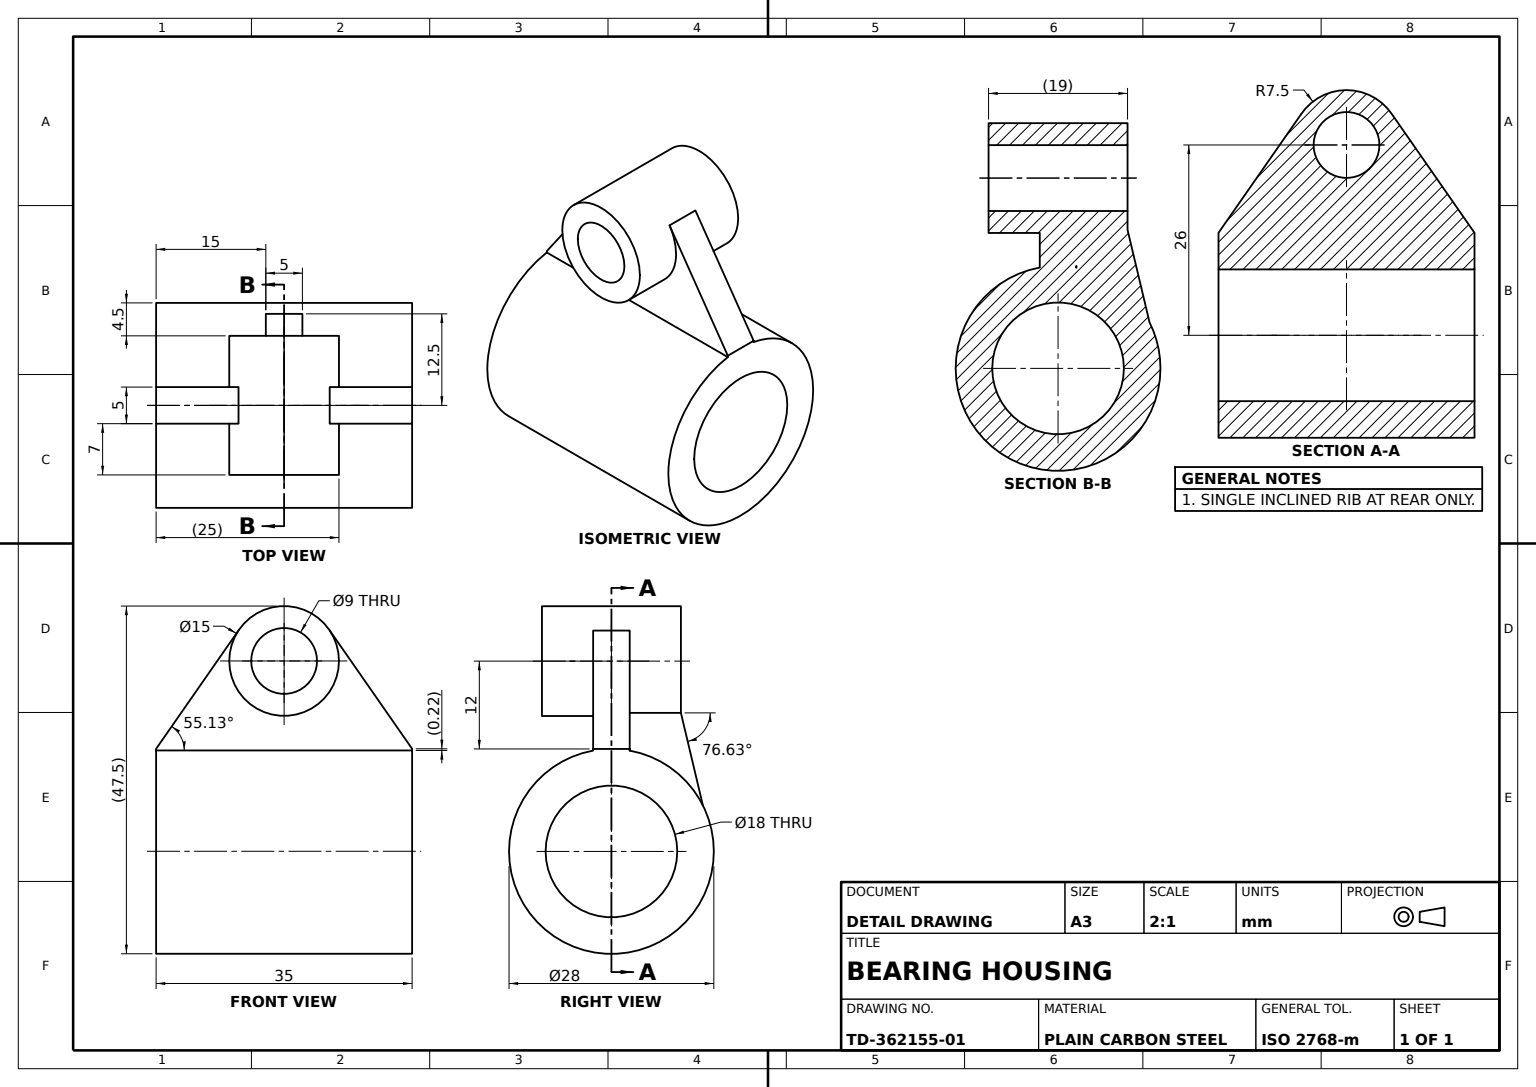
ISO-10303-21;
HEADER;
FILE_DESCRIPTION((''),'2;1');
FILE_NAME('','',(''),(''),'','','');
FILE_SCHEMA(('AUTOMOTIVE_DESIGN'));
ENDSEC;
DATA;
#1=APPLICATION_CONTEXT('');
#2=PRODUCT_CONTEXT('',#1,'mechanical');
#3=PRODUCT('','','',(#2));
#4=PRODUCT_DEFINITION_FORMATION('','',#3);
#5=PRODUCT_DEFINITION_CONTEXT('',#1,'design');
#6=PRODUCT_DEFINITION('','',#4,#5);
#7=PRODUCT_DEFINITION_SHAPE('','',#6);
#8=(LENGTH_UNIT()NAMED_UNIT(*)SI_UNIT(.MILLI.,.METRE.));
#9=(NAMED_UNIT(*)PLANE_ANGLE_UNIT()SI_UNIT($,.RADIAN.));
#10=(NAMED_UNIT(*)SI_UNIT($,.STERADIAN.)SOLID_ANGLE_UNIT());
#11=UNCERTAINTY_MEASURE_WITH_UNIT(LENGTH_MEASURE(1.E-05),#8,'distance_accuracy_value','');
#12=(GEOMETRIC_REPRESENTATION_CONTEXT(3)GLOBAL_UNCERTAINTY_ASSIGNED_CONTEXT((#11))GLOBAL_UNIT_ASSIGNED_CONTEXT((#8,#9,#10))REPRESENTATION_CONTEXT('',''));
#13=CARTESIAN_POINT('',(9.5,26.,-22.));
#14=VERTEX_POINT('',#13);
#15=CARTESIAN_POINT('',(9.5,26.,-13.));
#16=VERTEX_POINT('',#15);
#17=CARTESIAN_POINT('',(9.5,26.,-17.5));
#18=DIRECTION('',(1.,0.,0.));
#19=DIRECTION('',(0.,0.,-1.));
#20=AXIS2_PLACEMENT_3D('',#17,#18,#19);
#21=CIRCLE('',#20,4.5);
#22=EDGE_CURVE('',#14,#16,#21,.T.);
#23=ORIENTED_EDGE('',*,*,#22,.F.);
#24=EDGE_CURVE('',#16,#14,#21,.T.);
#25=ORIENTED_EDGE('',*,*,#24,.F.);
#26=EDGE_LOOP('',(#23,#25));
#27=FACE_BOUND('',#26,.T.);
#28=CARTESIAN_POINT('',(9.5,18.928932,-20.));
#29=VERTEX_POINT('',#28);
#30=CARTESIAN_POINT('',(9.5,18.928932,-15.));
#31=VERTEX_POINT('',#30);
#32=CARTESIAN_POINT('',(9.5,18.928932,-35.));
#33=DIRECTION('',(0.,0.,1.));
#34=VECTOR('',#33,1000.);
#35=LINE('',#32,#34);
#36=EDGE_CURVE('',#29,#31,#35,.T.);
#37=ORIENTED_EDGE('',*,*,#36,.F.);
#38=CARTESIAN_POINT('',(9.5,26.,-25.));
#39=VERTEX_POINT('',#38);
#40=CIRCLE('',#20,7.5);
#41=EDGE_CURVE('',#29,#39,#40,.T.);
#42=ORIENTED_EDGE('',*,*,#41,.T.);
#43=CARTESIAN_POINT('',(9.5,26.,-10.));
#44=VERTEX_POINT('',#43);
#45=EDGE_CURVE('',#39,#44,#40,.T.);
#46=ORIENTED_EDGE('',*,*,#45,.T.);
#47=EDGE_CURVE('',#44,#31,#40,.T.);
#48=ORIENTED_EDGE('',*,*,#47,.T.);
#49=EDGE_LOOP('',(#37,#42,#46,#48));
#50=FACE_OUTER_BOUND('',#49,.T.);
#51=PLANE('',#20);
#52=ADVANCED_FACE('',(#27,#50),#51,.T.);
#53=CARTESIAN_POINT('',(14.,0.,-35.));
#54=VERTEX_POINT('',#53);
#55=CARTESIAN_POINT('',(14.,0.,0.));
#56=VERTEX_POINT('',#55);
#57=LINE('',#53,#34);
#58=EDGE_CURVE('',#54,#56,#57,.T.);
#59=ORIENTED_EDGE('',*,*,#58,.T.);
#60=CARTESIAN_POINT('',(-14.,0.,0.));
#61=VERTEX_POINT('',#60);
#62=CARTESIAN_POINT('',(0.,0.,0.));
#63=AXIS2_PLACEMENT_3D('',#62,#33,#18);
#64=CIRCLE('',#63,14.);
#65=EDGE_CURVE('',#61,#56,#64,.T.);
#66=ORIENTED_EDGE('',*,*,#65,.F.);
#67=CARTESIAN_POINT('',(-14.,0.,-35.));
#68=VERTEX_POINT('',#67);
#69=LINE('',#67,#34);
#70=EDGE_CURVE('',#68,#61,#69,.T.);
#71=ORIENTED_EDGE('',*,*,#70,.F.);
#72=CARTESIAN_POINT('',(0.,0.,-35.));
#73=AXIS2_PLACEMENT_3D('',#72,#33,#18);
#74=CIRCLE('',#73,14.);
#75=EDGE_CURVE('',#68,#54,#74,.T.);
#76=ORIENTED_EDGE('',*,*,#75,.T.);
#77=EDGE_LOOP('',(#59,#66,#71,#76));
#78=FACE_OUTER_BOUND('',#77,.T.);
#79=CYLINDRICAL_SURFACE('',#73,14.);
#80=ADVANCED_FACE('',(#78),#79,.T.);
#81=CARTESIAN_POINT('',(2.5,26.,-25.));
#82=VERTEX_POINT('',#81);
#83=CARTESIAN_POINT('',(-2.5,26.,-25.));
#84=VECTOR('',#18,1000.);
#85=LINE('',#83,#84);
#86=EDGE_CURVE('',#82,#39,#85,.T.);
#87=ORIENTED_EDGE('',*,*,#86,.F.);
#88=CARTESIAN_POINT('',(2.5,30.172304,-23.732325));
#89=VERTEX_POINT('',#88);
#90=CARTESIAN_POINT('',(2.5,26.,-17.5));
#91=AXIS2_PLACEMENT_3D('',#90,#18,#19);
#92=CIRCLE('',#91,7.5);
#93=EDGE_CURVE('',#82,#89,#92,.T.);
#94=ORIENTED_EDGE('',*,*,#93,.T.);
#95=CARTESIAN_POINT('',(-2.5,30.172304,-23.732325));
#96=VERTEX_POINT('',#95);
#97=LINE('',#95,#84);
#98=EDGE_CURVE('',#96,#89,#97,.T.);
#99=ORIENTED_EDGE('',*,*,#98,.F.);
#100=VERTEX_POINT('',#83);
#101=CARTESIAN_POINT('',(-2.5,26.,-17.5));
#102=DIRECTION('',(-1.,0.,0.));
#103=AXIS2_PLACEMENT_3D('',#101,#102,#33);
#104=CIRCLE('',#103,7.5);
#105=EDGE_CURVE('',#96,#100,#104,.T.);
#106=ORIENTED_EDGE('',*,*,#105,.T.);
#107=CARTESIAN_POINT('',(-9.5,26.,-25.));
#108=VERTEX_POINT('',#107);
#109=EDGE_CURVE('',#108,#100,#85,.T.);
#110=ORIENTED_EDGE('',*,*,#109,.F.);
#111=CARTESIAN_POINT('',(-9.5,26.,-10.));
#112=VERTEX_POINT('',#111);
#113=CARTESIAN_POINT('',(-9.5,26.,-17.5));
#114=AXIS2_PLACEMENT_3D('',#113,#102,#33);
#115=CIRCLE('',#114,7.5);
#116=EDGE_CURVE('',#112,#108,#115,.T.);
#117=ORIENTED_EDGE('',*,*,#116,.F.);
#118=CARTESIAN_POINT('',(-2.5,26.,-10.));
#119=VERTEX_POINT('',#118);
#120=LINE('',#118,#84);
#121=EDGE_CURVE('',#112,#119,#120,.T.);
#122=ORIENTED_EDGE('',*,*,#121,.T.);
#123=CARTESIAN_POINT('',(-2.5,30.172304,-11.267675));
#124=VERTEX_POINT('',#123);
#125=EDGE_CURVE('',#119,#124,#104,.T.);
#126=ORIENTED_EDGE('',*,*,#125,.T.);
#127=CARTESIAN_POINT('',(2.5,30.172304,-11.267675));
#128=VERTEX_POINT('',#127);
#129=LINE('',#123,#84);
#130=EDGE_CURVE('',#124,#128,#129,.T.);
#131=ORIENTED_EDGE('',*,*,#130,.T.);
#132=CARTESIAN_POINT('',(2.5,26.,-10.));
#133=VERTEX_POINT('',#132);
#134=EDGE_CURVE('',#128,#133,#92,.T.);
#135=ORIENTED_EDGE('',*,*,#134,.T.);
#136=EDGE_CURVE('',#133,#44,#120,.T.);
#137=ORIENTED_EDGE('',*,*,#136,.T.);
#138=ORIENTED_EDGE('',*,*,#45,.F.);
#139=EDGE_LOOP('',(#87,#94,#99,#106,#110,#117,#122,#126,#131,#135,#137,#138));
#140=FACE_OUTER_BOUND('',#139,.T.);
#141=AXIS2_PLACEMENT_3D('',#101,#18,#19);
#142=CYLINDRICAL_SURFACE('',#141,7.5);
#143=ADVANCED_FACE('',(#140),#142,.T.);
#144=CARTESIAN_POINT('',(2.5,18.928932,-20.));
#145=VERTEX_POINT('',#144);
#146=CARTESIAN_POINT('',(2.5,14.,-20.));
#147=VERTEX_POINT('',#146);
#148=DIRECTION('',(0.,-1.,0.));
#149=VECTOR('',#148,1000.);
#150=LINE('',#144,#149);
#151=EDGE_CURVE('',#145,#147,#150,.T.);
#152=ORIENTED_EDGE('',*,*,#151,.F.);
#153=VECTOR('',#102,1000.);
#154=LINE('',#28,#153);
#155=EDGE_CURVE('',#29,#145,#154,.T.);
#156=ORIENTED_EDGE('',*,*,#155,.F.);
#157=CARTESIAN_POINT('',(12.502197,6.300402,-20.));
#158=VERTEX_POINT('',#157);
#159=DIRECTION('',(-0.231285455,0.972885933,0.));
#160=VECTOR('',#159,1000.);
#161=LINE('',#28,#160);
#162=EDGE_CURVE('',#158,#29,#161,.T.);
#163=ORIENTED_EDGE('',*,*,#162,.F.);
#164=CARTESIAN_POINT('',(2.5,13.774977,-20.));
#165=VERTEX_POINT('',#164);
#166=CARTESIAN_POINT('',(0.,0.,-20.));
#167=AXIS2_PLACEMENT_3D('',#166,#19,#18);
#168=CIRCLE('',#167,14.);
#169=EDGE_CURVE('',#165,#158,#168,.T.);
#170=ORIENTED_EDGE('',*,*,#169,.F.);
#171=EDGE_CURVE('',#147,#165,#150,.T.);
#172=ORIENTED_EDGE('',*,*,#171,.F.);
#173=EDGE_LOOP('',(#152,#156,#163,#170,#172));
#174=FACE_OUTER_BOUND('',#173,.T.);
#175=AXIS2_PLACEMENT_3D('',#166,#33,#18);
#176=PLANE('',#175);
#177=ADVANCED_FACE('',(#174),#176,.F.);
#178=CARTESIAN_POINT('',(2.5,13.774977,-15.));
#179=VERTEX_POINT('',#178);
#180=CARTESIAN_POINT('',(12.502197,6.300402,-15.));
#181=VERTEX_POINT('',#180);
#182=CARTESIAN_POINT('',(0.,0.,-15.));
#183=AXIS2_PLACEMENT_3D('',#182,#19,#18);
#184=CIRCLE('',#183,14.);
#185=EDGE_CURVE('',#179,#181,#184,.T.);
#186=ORIENTED_EDGE('',*,*,#185,.T.);
#187=LINE('',#30,#160);
#188=EDGE_CURVE('',#181,#31,#187,.T.);
#189=ORIENTED_EDGE('',*,*,#188,.T.);
#190=CARTESIAN_POINT('',(2.5,18.928932,-15.));
#191=VERTEX_POINT('',#190);
#192=LINE('',#190,#153);
#193=EDGE_CURVE('',#31,#191,#192,.T.);
#194=ORIENTED_EDGE('',*,*,#193,.T.);
#195=CARTESIAN_POINT('',(2.5,14.,-15.));
#196=VERTEX_POINT('',#195);
#197=LINE('',#190,#149);
#198=EDGE_CURVE('',#191,#196,#197,.T.);
#199=ORIENTED_EDGE('',*,*,#198,.T.);
#200=EDGE_CURVE('',#196,#179,#197,.T.);
#201=ORIENTED_EDGE('',*,*,#200,.T.);
#202=EDGE_LOOP('',(#186,#189,#194,#199,#201));
#203=FACE_OUTER_BOUND('',#202,.T.);
#204=AXIS2_PLACEMENT_3D('',#182,#33,#18);
#205=PLANE('',#204);
#206=ADVANCED_FACE('',(#203),#205,.T.);
#207=EDGE_CURVE('',#145,#82,#92,.T.);
#208=ORIENTED_EDGE('',*,*,#207,.F.);
#209=ORIENTED_EDGE('',*,*,#151,.T.);
#210=CARTESIAN_POINT('',(2.5,14.,-35.));
#211=VERTEX_POINT('',#210);
#212=LINE('',#210,#34);
#213=EDGE_CURVE('',#211,#147,#212,.T.);
#214=ORIENTED_EDGE('',*,*,#213,.F.);
#215=CARTESIAN_POINT('',(2.5,20.991542,-30.128807));
#216=DIRECTION('',(0.,0.820491715,0.571658417));
#217=VECTOR('',#216,1000.);
#218=LINE('',#215,#217);
#219=EDGE_CURVE('',#211,#89,#218,.T.);
#220=ORIENTED_EDGE('',*,*,#219,.T.);
#221=ORIENTED_EDGE('',*,*,#93,.F.);
#222=EDGE_LOOP('',(#208,#209,#214,#220,#221));
#223=FACE_OUTER_BOUND('',#222,.T.);
#224=CARTESIAN_POINT('',(2.5,0.,0.));
#225=AXIS2_PLACEMENT_3D('',#224,#18,#19);
#226=PLANE('',#225);
#227=ADVANCED_FACE('',(#223),#226,.T.);
#228=ORIENTED_EDGE('',*,*,#171,.T.);
#229=CARTESIAN_POINT('',(2.5,13.774977,-35.));
#230=LINE('',#229,#34);
#231=EDGE_CURVE('',#165,#179,#230,.T.);
#232=ORIENTED_EDGE('',*,*,#231,.T.);
#233=ORIENTED_EDGE('',*,*,#200,.F.);
#234=EDGE_CURVE('',#147,#196,#212,.T.);
#235=ORIENTED_EDGE('',*,*,#234,.F.);
#236=EDGE_LOOP('',(#228,#232,#233,#235));
#237=FACE_OUTER_BOUND('',#236,.T.);
#238=CARTESIAN_POINT('',(2.5,18.928932,-35.));
#239=AXIS2_PLACEMENT_3D('',#238,#102,#33);
#240=PLANE('',#239);
#241=ADVANCED_FACE('',(#237),#240,.T.);
#242=CARTESIAN_POINT('',(2.495507,13.775792,0.));
#243=VERTEX_POINT('',#242);
#244=CARTESIAN_POINT('',(2.5,14.,0.));
#245=VERTEX_POINT('',#244);
#246=CARTESIAN_POINT('',(2.218565,-0.044458,0.));
#247=DIRECTION('',(0.020034845,0.999799282,0.));
#248=VECTOR('',#247,1000.);
#249=LINE('',#246,#248);
#250=EDGE_CURVE('',#243,#245,#249,.T.);
#251=ORIENTED_EDGE('',*,*,#250,.F.);
#252=CARTESIAN_POINT('',(2.495507,13.775792,-35.));
#253=VERTEX_POINT('',#252);
#254=LINE('',#252,#34);
#255=EDGE_CURVE('',#253,#243,#254,.T.);
#256=ORIENTED_EDGE('',*,*,#255,.F.);
#257=CARTESIAN_POINT('',(2.218565,-0.044458,-35.));
#258=LINE('',#257,#248);
#259=EDGE_CURVE('',#253,#211,#258,.T.);
#260=ORIENTED_EDGE('',*,*,#259,.T.);
#261=ORIENTED_EDGE('',*,*,#213,.T.);
#262=ORIENTED_EDGE('',*,*,#234,.T.);
#263=EDGE_CURVE('',#196,#245,#212,.T.);
#264=ORIENTED_EDGE('',*,*,#263,.T.);
#265=EDGE_LOOP('',(#251,#256,#260,#261,#262,#264));
#266=FACE_OUTER_BOUND('',#265,.T.);
#267=DIRECTION('',(0.999799282,-0.020034845,0.));
#268=AXIS2_PLACEMENT_3D('',#257,#267,#247);
#269=PLANE('',#268);
#270=ADVANCED_FACE('',(#266),#269,.T.);
#271=ORIENTED_EDGE('',*,*,#47,.F.);
#272=ORIENTED_EDGE('',*,*,#136,.F.);
#273=EDGE_CURVE('',#133,#191,#92,.T.);
#274=ORIENTED_EDGE('',*,*,#273,.T.);
#275=ORIENTED_EDGE('',*,*,#193,.F.);
#276=EDGE_LOOP('',(#271,#272,#274,#275));
#277=FACE_OUTER_BOUND('',#276,.T.);
#278=ADVANCED_FACE('',(#277),#142,.T.);
#279=CARTESIAN_POINT('',(-2.5,13.774977,-35.));
#280=VERTEX_POINT('',#279);
#281=EDGE_CURVE('',#280,#68,#74,.T.);
#282=ORIENTED_EDGE('',*,*,#281,.T.);
#283=ORIENTED_EDGE('',*,*,#70,.T.);
#284=CARTESIAN_POINT('',(-2.5,13.774977,0.));
#285=VERTEX_POINT('',#284);
#286=EDGE_CURVE('',#285,#61,#64,.T.);
#287=ORIENTED_EDGE('',*,*,#286,.F.);
#288=LINE('',#279,#34);
#289=EDGE_CURVE('',#280,#285,#288,.T.);
#290=ORIENTED_EDGE('',*,*,#289,.F.);
#291=EDGE_LOOP('',(#282,#283,#287,#290));
#292=FACE_OUTER_BOUND('',#291,.T.);
#293=ADVANCED_FACE('',(#292),#79,.T.);
#294=CARTESIAN_POINT('',(-9.5,26.,-22.));
#295=VERTEX_POINT('',#294);
#296=CARTESIAN_POINT('',(-40.5,26.,-22.));
#297=LINE('',#296,#84);
#298=EDGE_CURVE('',#295,#14,#297,.T.);
#299=ORIENTED_EDGE('',*,*,#298,.T.);
#300=ORIENTED_EDGE('',*,*,#22,.T.);
#301=CARTESIAN_POINT('',(-9.5,26.,-13.));
#302=VERTEX_POINT('',#301);
#303=CARTESIAN_POINT('',(-40.5,26.,-13.));
#304=LINE('',#303,#84);
#305=EDGE_CURVE('',#302,#16,#304,.T.);
#306=ORIENTED_EDGE('',*,*,#305,.F.);
#307=CIRCLE('',#114,4.5);
#308=EDGE_CURVE('',#302,#295,#307,.T.);
#309=ORIENTED_EDGE('',*,*,#308,.T.);
#310=EDGE_LOOP('',(#299,#300,#306,#309));
#311=FACE_OUTER_BOUND('',#310,.T.);
#312=CARTESIAN_POINT('',(-40.5,26.,-17.5));
#313=AXIS2_PLACEMENT_3D('',#312,#18,#19);
#314=CYLINDRICAL_SURFACE('',#313,4.5);
#315=ADVANCED_FACE('',(#311),#314,.F.);
#316=EDGE_CURVE('',#100,#119,#104,.T.);
#317=ORIENTED_EDGE('',*,*,#316,.T.);
#318=ORIENTED_EDGE('',*,*,#121,.F.);
#319=EDGE_CURVE('',#108,#112,#115,.T.);
#320=ORIENTED_EDGE('',*,*,#319,.F.);
#321=ORIENTED_EDGE('',*,*,#109,.T.);
#322=EDGE_LOOP('',(#317,#318,#320,#321));
#323=FACE_OUTER_BOUND('',#322,.T.);
#324=ADVANCED_FACE('',(#323),#142,.T.);
#325=CARTESIAN_POINT('',(2.5,4.575107,6.566574));
#326=DIRECTION('',(0.,0.820491715,-0.571658417));
#327=VECTOR('',#326,1000.);
#328=LINE('',#325,#327);
#329=EDGE_CURVE('',#245,#128,#328,.T.);
#330=ORIENTED_EDGE('',*,*,#329,.F.);
#331=ORIENTED_EDGE('',*,*,#263,.F.);
#332=ORIENTED_EDGE('',*,*,#198,.F.);
#333=ORIENTED_EDGE('',*,*,#273,.F.);
#334=ORIENTED_EDGE('',*,*,#134,.F.);
#335=EDGE_LOOP('',(#330,#331,#332,#333,#334));
#336=FACE_OUTER_BOUND('',#335,.T.);
#337=ADVANCED_FACE('',(#336),#226,.T.);
#338=CARTESIAN_POINT('',(-9.,0.,-35.));
#339=VERTEX_POINT('',#338);
#340=CARTESIAN_POINT('',(-9.,0.,0.));
#341=VERTEX_POINT('',#340);
#342=LINE('',#338,#34);
#343=EDGE_CURVE('',#339,#341,#342,.T.);
#344=ORIENTED_EDGE('',*,*,#343,.F.);
#345=CARTESIAN_POINT('',(9.,0.,-35.));
#346=VERTEX_POINT('',#345);
#347=CIRCLE('',#73,9.);
#348=EDGE_CURVE('',#346,#339,#347,.T.);
#349=ORIENTED_EDGE('',*,*,#348,.F.);
#350=CARTESIAN_POINT('',(9.,0.,0.));
#351=VERTEX_POINT('',#350);
#352=LINE('',#345,#34);
#353=EDGE_CURVE('',#346,#351,#352,.T.);
#354=ORIENTED_EDGE('',*,*,#353,.T.);
#355=CIRCLE('',#63,9.);
#356=EDGE_CURVE('',#351,#341,#355,.T.);
#357=ORIENTED_EDGE('',*,*,#356,.T.);
#358=EDGE_LOOP('',(#344,#349,#354,#357));
#359=FACE_OUTER_BOUND('',#358,.T.);
#360=CYLINDRICAL_SURFACE('',#73,9.);
#361=ADVANCED_FACE('',(#359),#360,.F.);
#362=EDGE_CURVE('',#341,#351,#355,.T.);
#363=ORIENTED_EDGE('',*,*,#362,.T.);
#364=ORIENTED_EDGE('',*,*,#353,.F.);
#365=EDGE_CURVE('',#339,#346,#347,.T.);
#366=ORIENTED_EDGE('',*,*,#365,.F.);
#367=ORIENTED_EDGE('',*,*,#343,.T.);
#368=EDGE_LOOP('',(#363,#364,#366,#367));
#369=FACE_OUTER_BOUND('',#368,.T.);
#370=ADVANCED_FACE('',(#369),#360,.F.);
#371=ORIENTED_EDGE('',*,*,#116,.T.);
#372=ORIENTED_EDGE('',*,*,#319,.T.);
#373=EDGE_LOOP('',(#371,#372));
#374=FACE_OUTER_BOUND('',#373,.T.);
#375=ORIENTED_EDGE('',*,*,#308,.F.);
#376=EDGE_CURVE('',#295,#302,#307,.T.);
#377=ORIENTED_EDGE('',*,*,#376,.F.);
#378=EDGE_LOOP('',(#375,#377));
#379=FACE_BOUND('',#378,.T.);
#380=PLANE('',#114);
#381=ADVANCED_FACE('',(#374,#379),#380,.T.);
#382=ORIENTED_EDGE('',*,*,#155,.T.);
#383=ORIENTED_EDGE('',*,*,#207,.T.);
#384=ORIENTED_EDGE('',*,*,#86,.T.);
#385=ORIENTED_EDGE('',*,*,#41,.F.);
#386=EDGE_LOOP('',(#382,#383,#384,#385));
#387=FACE_OUTER_BOUND('',#386,.T.);
#388=ADVANCED_FACE('',(#387),#142,.T.);
#389=CARTESIAN_POINT('',(12.502197,6.300402,-35.));
#390=LINE('',#389,#34);
#391=EDGE_CURVE('',#158,#181,#390,.T.);
#392=ORIENTED_EDGE('',*,*,#391,.T.);
#393=ORIENTED_EDGE('',*,*,#185,.F.);
#394=ORIENTED_EDGE('',*,*,#231,.F.);
#395=ORIENTED_EDGE('',*,*,#169,.T.);
#396=EDGE_LOOP('',(#392,#393,#394,#395));
#397=FACE_BOUND('',#396,.T.);
#398=ORIENTED_EDGE('',*,*,#255,.T.);
#399=EDGE_CURVE('',#56,#243,#64,.T.);
#400=ORIENTED_EDGE('',*,*,#399,.F.);
#401=ORIENTED_EDGE('',*,*,#58,.F.);
#402=EDGE_CURVE('',#54,#253,#74,.T.);
#403=ORIENTED_EDGE('',*,*,#402,.T.);
#404=EDGE_LOOP('',(#398,#400,#401,#403));
#405=FACE_OUTER_BOUND('',#404,.T.);
#406=ADVANCED_FACE('',(#397,#405),#79,.T.);
#407=ORIENTED_EDGE('',*,*,#316,.F.);
#408=ORIENTED_EDGE('',*,*,#105,.F.);
#409=CARTESIAN_POINT('',(-2.5,14.,-35.));
#410=VERTEX_POINT('',#409);
#411=CARTESIAN_POINT('',(-2.5,20.991542,-30.128807));
#412=LINE('',#411,#217);
#413=EDGE_CURVE('',#410,#96,#412,.T.);
#414=ORIENTED_EDGE('',*,*,#413,.F.);
#415=CARTESIAN_POINT('',(-2.5,0.,-35.));
#416=LINE('',#415,#149);
#417=EDGE_CURVE('',#410,#280,#416,.T.);
#418=ORIENTED_EDGE('',*,*,#417,.T.);
#419=ORIENTED_EDGE('',*,*,#289,.T.);
#420=CARTESIAN_POINT('',(-2.5,14.,0.));
#421=VERTEX_POINT('',#420);
#422=CARTESIAN_POINT('',(-2.5,0.,0.));
#423=LINE('',#422,#149);
#424=EDGE_CURVE('',#421,#285,#423,.T.);
#425=ORIENTED_EDGE('',*,*,#424,.F.);
#426=CARTESIAN_POINT('',(-2.5,4.575107,6.566574));
#427=LINE('',#426,#327);
#428=EDGE_CURVE('',#421,#124,#427,.T.);
#429=ORIENTED_EDGE('',*,*,#428,.T.);
#430=ORIENTED_EDGE('',*,*,#125,.F.);
#431=EDGE_LOOP('',(#407,#408,#414,#418,#419,#425,#429,#430));
#432=FACE_OUTER_BOUND('',#431,.T.);
#433=AXIS2_PLACEMENT_3D('',#422,#18,#19);
#434=PLANE('',#433);
#435=ADVANCED_FACE('',(#432),#434,.F.);
#436=ORIENTED_EDGE('',*,*,#298,.F.);
#437=ORIENTED_EDGE('',*,*,#376,.T.);
#438=ORIENTED_EDGE('',*,*,#305,.T.);
#439=ORIENTED_EDGE('',*,*,#24,.T.);
#440=EDGE_LOOP('',(#436,#437,#438,#439));
#441=FACE_OUTER_BOUND('',#440,.T.);
#442=ADVANCED_FACE('',(#441),#314,.F.);
#443=CARTESIAN_POINT('',(0.,14.,-35.));
#444=LINE('',#443,#153);
#445=EDGE_CURVE('',#211,#410,#444,.T.);
#446=ORIENTED_EDGE('',*,*,#445,.F.);
#447=ORIENTED_EDGE('',*,*,#259,.F.);
#448=ORIENTED_EDGE('',*,*,#402,.F.);
#449=ORIENTED_EDGE('',*,*,#75,.F.);
#450=ORIENTED_EDGE('',*,*,#281,.F.);
#451=ORIENTED_EDGE('',*,*,#417,.F.);
#452=EDGE_LOOP('',(#446,#447,#448,#449,#450,#451));
#453=FACE_OUTER_BOUND('',#452,.T.);
#454=ORIENTED_EDGE('',*,*,#348,.T.);
#455=ORIENTED_EDGE('',*,*,#365,.T.);
#456=EDGE_LOOP('',(#454,#455));
#457=FACE_BOUND('',#456,.T.);
#458=PLANE('',#73);
#459=ADVANCED_FACE('',(#453,#457),#458,.F.);
#460=ORIENTED_EDGE('',*,*,#413,.T.);
#461=ORIENTED_EDGE('',*,*,#98,.T.);
#462=ORIENTED_EDGE('',*,*,#219,.F.);
#463=ORIENTED_EDGE('',*,*,#445,.T.);
#464=EDGE_LOOP('',(#460,#461,#462,#463));
#465=FACE_OUTER_BOUND('',#464,.T.);
#466=DIRECTION('',(0.,0.571658417,-0.820491715));
#467=AXIS2_PLACEMENT_3D('',#411,#466,#216);
#468=PLANE('',#467);
#469=ADVANCED_FACE('',(#465),#468,.T.);
#470=ORIENTED_EDGE('',*,*,#162,.T.);
#471=ORIENTED_EDGE('',*,*,#36,.T.);
#472=ORIENTED_EDGE('',*,*,#188,.F.);
#473=ORIENTED_EDGE('',*,*,#391,.F.);
#474=EDGE_LOOP('',(#470,#471,#472,#473));
#475=FACE_OUTER_BOUND('',#474,.T.);
#476=DIRECTION('',(0.972885933,0.231285455,0.));
#477=AXIS2_PLACEMENT_3D('',#32,#476,#159);
#478=PLANE('',#477);
#479=ADVANCED_FACE('',(#475),#478,.T.);
#480=ORIENTED_EDGE('',*,*,#362,.F.);
#481=ORIENTED_EDGE('',*,*,#356,.F.);
#482=EDGE_LOOP('',(#480,#481));
#483=FACE_BOUND('',#482,.T.);
#484=ORIENTED_EDGE('',*,*,#65,.T.);
#485=ORIENTED_EDGE('',*,*,#399,.T.);
#486=ORIENTED_EDGE('',*,*,#250,.T.);
#487=CARTESIAN_POINT('',(0.,14.,0.));
#488=LINE('',#487,#153);
#489=EDGE_CURVE('',#245,#421,#488,.T.);
#490=ORIENTED_EDGE('',*,*,#489,.T.);
#491=ORIENTED_EDGE('',*,*,#424,.T.);
#492=ORIENTED_EDGE('',*,*,#286,.T.);
#493=EDGE_LOOP('',(#484,#485,#486,#490,#491,#492));
#494=FACE_OUTER_BOUND('',#493,.T.);
#495=PLANE('',#63);
#496=ADVANCED_FACE('',(#483,#494),#495,.T.);
#497=ORIENTED_EDGE('',*,*,#489,.F.);
#498=ORIENTED_EDGE('',*,*,#329,.T.);
#499=ORIENTED_EDGE('',*,*,#130,.F.);
#500=ORIENTED_EDGE('',*,*,#428,.F.);
#501=EDGE_LOOP('',(#497,#498,#499,#500));
#502=FACE_OUTER_BOUND('',#501,.T.);
#503=DIRECTION('',(0.,-0.571658417,-0.820491715));
#504=AXIS2_PLACEMENT_3D('',#426,#503,#326);
#505=PLANE('',#504);
#506=ADVANCED_FACE('',(#502),#505,.F.);
#507=CLOSED_SHELL('',(#52,#80,#143,#177,#206,#227,#241,#270,#278,#293,#315,#324,#337,#361,#370,#381,#388,#406,#435,#442,#459,#469,#479,#496,#506));
#508=MANIFOLD_SOLID_BREP('',#507);
#509=ADVANCED_BREP_SHAPE_REPRESENTATION('',(#508),#12);
#510=SHAPE_DEFINITION_REPRESENTATION(#7,#509);
ENDSEC;
END-ISO-10303-21;
